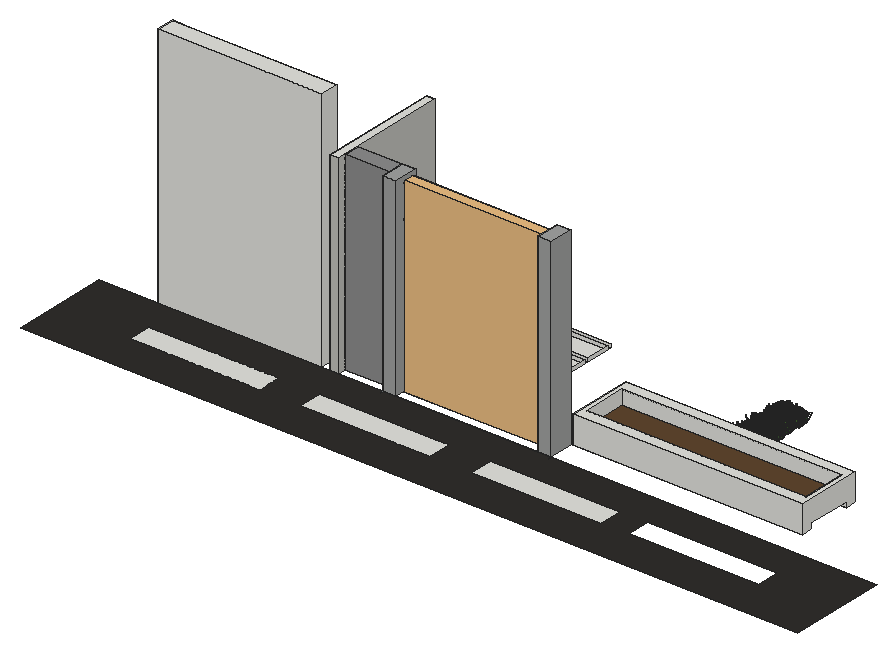
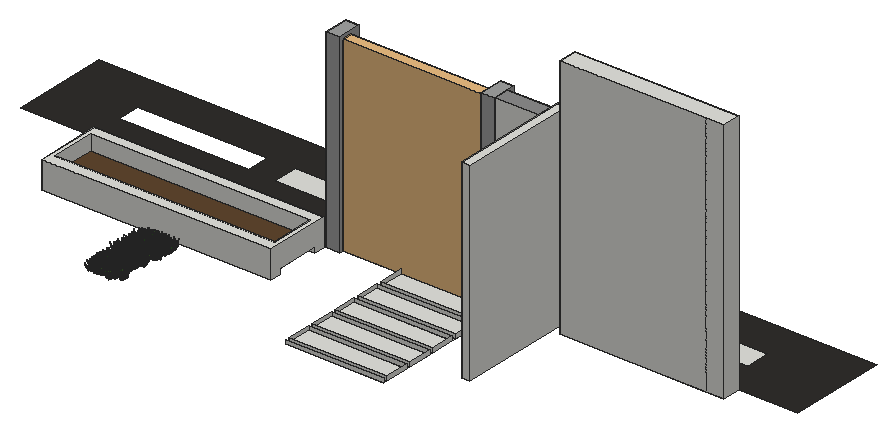
# SketchUp Ruby script. Lengths in inches.
U = 1.inch
M = Sketchup.active_model
def pt(a) = Geom::Point3d.new(a.map { |v| v * U })
def face(e, loops, mat)
  f = e.add_face(loops[0].map { |a| pt(a) })
  loops[1..].each { |l| e.add_face(l.map { |a| pt(a) }).erase! }
  f.material = f.back_material = mat if mat
  f
end
# faces: each face lists its corners as indices into pts; further lists are holes
def faces(e, pts, list, mat = nil) = list.each { |f| face(e, (f[0].is_a?(Array) ? f : [f]).map { |l| l.map { |i| pts[i] } }, mat) }
# xy, xz, yz: faces in a plane at the given z, y or x. An outline is a flat list of corners, or four numbers for a rectangle; further outlines are holes
def ring(l) = l.size == 4 ? [[l[0], l[1]], [l[2], l[1]], [l[2], l[3]], [l[0], l[3]]] : l.each_slice(2).to_a
def flat(e, list, mat, &to3) = list.each { |f| face(e, (f[0].is_a?(Array) ? f : [f]).map { |l| ring(l).map { |u, v| to3.(u, v) } }, mat) }
def xy(e, z, list, mat = nil) = flat(e, list, mat) { |x, y| [x, y, z] }
def xz(e, y, list, mat = nil) = flat(e, list, mat) { |x, z| [x, y, z] }
def yz(e, x, list, mat = nil) = flat(e, list, mat) { |y, z| [x, y, z] }
def lines(e, pts, list) = list.each { |a, b| e.add_line(pt(pts[a]), pt(pts[b])) }
# prism: a flat outline (further loops are holes) pulled along v
def prism(e, loops, v, mat = nil)
  f = face(e, loops, mat); d = Geom::Vector3d.new(v.map { |x| x * U })
  f.pushpull(f.normal.samedirection?(d) ? d.length : -d.length)
end
def box(e, o, s, mat = nil) = prism(e, [[o, [o[0] + s[0], o[1], o[2]], [o[0] + s[0], o[1] + s[1], o[2]], [o[0], o[1] + s[1], o[2]]]], [0, 0, s[2]], mat)
def at(x, y, z, deg = 0) = Geom::Transformation.translation(pt([x, y, z])) * Geom::Transformation.rotation(ORIGIN, Z_AXIS, deg.degrees)
def axes(o, x, y, z) = Geom::Transformation.new([*x, 0, *y, 0, *z, 0, *pt(o).to_a, 1])
def part(name) = M.definitions.add(name)
# library, detail: a bought-in or finely detailed component or shape, given as its bounding box
def library(name, o, s) = part(name).tap { |d| box(d.entities, o, s) }
def detail(e, o, s) = box(e.add_group.entities, o, s)
def put(e, d, t, mat = nil) = e.add_instance(d, t).tap { |i| i.material = mat if mat }
def group(e, t, mat = nil) = e.add_group.tap { |g| g.transformation = t; g.material = mat if mat }.entities
root = M.entities
M.materials.add("18776129-polished-granite-texture-in-whites-grays-and-blacks").color = [192, 192, 186]
M.materials.add("Lisanne_Eraser").color = [146, 152, 155]
M.materials.add("Material1").color = [58, 110, 58]
M.materials.add("Material10").color = [48, 100, 38]
M.materials.add("Material3").color = [68, 110, 58]
M.materials.add("Material4").color = [48, 90, 38]
M.materials.add("Material5").color = [68, 110, 48]
M.materials.add("Material6").color = [48, 90, 48]
M.materials.add("Material8").color = [58, 90, 38]
M.materials.add("Material9").color = [68, 100, 58]
M.materials.add("Material__1").color = [95, 70, 46]
M.materials.add("Stone_A_200cmgach trang tri").color = [160, 161, 160]
M.materials.add("ThomThom - Hat1").color = [48, 46, 44]
M.materials.add("da-to-ong-xam").color = [140, 140, 140]
c1 = part("Group\#69")
xy(c1.entities,0,[[0,0,48,2]])
c2 = library("Group\#91",[0,0,0],[127.95,5.19,98.43])
c3 = part("grass00")
p = [[-0.6875,0.15,0],[-0.56,0.08,5.52],[-0.04,0.03,2.76],[0.48,-0.02,0],[0.35,-0.02,5.52],[-0.1,-0.14,5.52],
  [-0.12,0.65,8.37],[-0.42,0.65,8.37]]
faces(c3.entities,p,[[0,1,2,3],[3,2,4],[1,5,2],[5,4,2],[1,6,5],[4,5,6],[7,6,1]])
c4 = part("Group16\#1")
put(c4.entities,c3,axes([1.44,-0.61,-0.01],[0.05352,0.12609,0],[-0.10704,0.04543,0.07239],[0.06664,-0.02828,0.11628]),"Material6")
put(c4.entities,c3,axes([0.76,-0.15,-0.01],[0.04676,0.24062,0],[-0.23162,0.04501,0.06642],[0.0652,-0.01267,0.23595]),"Material3")
put(c4.entities,c3,axes([0.79,0.01,-0.01],[-0.00606,0.34651,0],[-0.34381,-0.00602,0.0432],[0.04319,0.00076,0.34386]))
put(c4.entities,c3,axes([1,0.23,-0.01],[-0.07192,0.31144,0],[-0.28722,-0.06632,0.1236],[0.12043,0.02781,0.29478]),"Material5")
put(c4.entities,c3,axes([1.66,0.77,-0.01],[-0.13828,0.29651,0],[-0.21551,-0.1005,0.22471],[0.20365,0.09498,0.23779]),"Material10")
put(c4.entities,c3,axes([0.6875,0.52,-0.01],[-0.18126,0.24051,0],[-0.22746,-0.17142,0.09788],[0.07817,0.05891,0.28481]),"Material5")
put(c4.entities,c3,axes([0.68,0.78,-0.01],[-0.215,0.18688,0],[-0.12385,-0.14248,0.21334],[0.13995,0.16101,0.18878]),"Material3")
put(c4.entities,c3,axes([0.56,1,-0.01],[-0.13756,0.07624,0],[-0.06159,-0.11112,0.0927],[0.04494,0.08108,0.12705]),"Material5")
put(c4.entities,c3,axes([0.2,0.64,-0.01],[-0.23729,0.07254,0],[-0.05711,-0.18681,0.153],[0.04473,0.14632,0.19535]),"Material10")
put(c4.entities,c3,axes([0.0625,0.72,-0.01],[-0.28874,0.02525,0],[-0.02179,-0.24916,0.14647],[0.01276,0.14591,0.25012]),"Material3")
put(c4.entities,c3,axes([-0.08,0.62,-0.01],[-0.34089,-0.04187,0],[0.03255,-0.26504,0.216],[-0.02633,0.21439,0.26703]),"Material10")
put(c4.entities,c3,axes([-0.34,0.98,-0.01],[-0.14314,-0.0493,0],[0.04397,-0.12769,0.06843],[-0.02228,0.0647,0.13505]),"Material10")
put(c4.entities,c3,axes([-0.87,1.45,-0.01],[-0.23488,-0.14114,0],[0.13761,-0.22901,0.06087],[-0.03135,0.05217,0.26717]))
put(c4.entities,c3,axes([-0.72,0.77,-0.01],[-0.14208,-0.13251,0],[0.07209,-0.0773,0.16301],[-0.11118,0.11922,0.1057]),"Material10")
put(c4.entities,c3,axes([-0.62,0.43,-0.01],[-0.14845,-0.21203,0],[0.18654,-0.13061,0.12304],[-0.10079,0.07057,0.22772]),"Material3")
put(c4.entities,c3,axes([-0.68,0.29,-0.01],[-0.13639,-0.32136,0],[0.31723,-0.13464,0.05579],[-0.05136,0.0218,0.34462]),"Material4")
put(c4.entities,c3,axes([-0.64,0.125,-0.01],[-0.0458,-0.23569,0],[0.22124,-0.043,0.08276],[-0.08124,0.01579,0.22538]),"Material1")
put(c4.entities,c3,axes([-1.6,-0.03,-0.01],[0.00576,-0.32897,0],[0.27526,0.00482,0.18018],[-0.18015,-0.00315,0.2753]),"Material5")
put(c4.entities,c3,axes([-1.36,-0.31,-0.01],[0.05718,-0.24765,0],[0.18172,0.04196,0.17267],[-0.16825,-0.03885,0.1865]),"Material10")
put(c4.entities,c3,axes([-1.54,-0.72,-0.01],[0.06537,-0.14017,0],[0.13555,0.06321,0.03939],[-0.0357,-0.01665,0.14956]))
put(c4.entities,c3,axes([-1.19,-0.9,-0.01],[0.09597,-0.12735,0],[0.11214,0.08451,0.07557],[-0.06035,-0.04548,0.14042]),"Material9")
put(c4.entities,c3,axes([-0.47,-0.54,-0.01],[0.11588,-0.10072,0],[0.0618,0.0711,0.12124],[-0.07953,-0.0915,0.0942]))
put(c4.entities,c3,axes([-0.47,-0.84,-0.01],[0.11927,-0.0661,0],[0.06603,0.11913,0.00646],[-0.00313,-0.00565,0.13621]),"Material5")
put(c4.entities,c3,axes([-0.38,-1.24,-0.01],[0.28037,-0.08571,0],[0.0618,0.20215,0.20315],[-0.05939,-0.19428,0.21139]),"Material9")
put(c4.entities,c3,axes([-0.06,-0.66,-0.01],[0.22719,-0.01987,0],[0.01247,0.14255,0.17758],[-0.01547,-0.17691,0.1431]),"Material8")
put(c4.entities,c3,axes([0.11,-0.89,-0.01],[0.14882,0.01828,0],[-0.01058,0.08611,0.12229],[0.01491,-0.12138,0.08676]),"Material6")
put(c4.entities,c3,axes([0.25,-0.72,-0.01],[0.20481,0.07053,0],[-0.06206,0.18022,0.10291],[0.03351,-0.0973,0.1906]),"Material6")
put(c4.entities,c3,axes([0.85,-1.42,-0.01],[0.16481,0.09904,0],[-0.09472,0.15762,0.05616],[0.02893,-0.04814,0.18389]),"Material5")
put(c4.entities,c3,axes([1.01,-1.09,-0.01],[0.21858,0.20385,0],[-0.17495,0.1876,0.15339],[0.10462,-0.11218,0.25652]),"Material10")
put(c4.entities,c3,axes([1.01,-0.71,-0.01],[0.08733,0.12473,0],[-0.06445,0.04512,0.13037],[0.1068,-0.07477,0.07867]),"Material6")
c5 = part("Group15\#1")
put(c5.entities,c4,at(0,0,0))
c6 = part("3darcstudiotree_grass00\#1")
put(c6.entities,c5,at(0,0,0))
xy(root,0,[[38.03,19.38,101.65,31.39],[121.5,19.38,185.12,31.39],[205.3,19.38,268.91,31.39],[138.47,57,186.47,70.5],[138.47,72.5,186.47,84.5],
  [138.47,86.5,186.47,98.5],[138.47,100.5,186.47,112.5],[138.47,114.5,186.47,126.5]])
xy(root,0,[[[0,0,380.77,48],[282.38,19.38,346,31.39],[38.03,19.38,101.65,31.39],[205.3,19.38,268.91,31.39],[121.5,19.38,185.12,31.39]]],"ThomThom - Hat1")
xz(root,57,[[138.47,0,186.47,2]])
xz(root,70.5,[[138.47,0,186.47,2]])
xz(root,72.5,[[138.47,0,186.47,2]])
xz(root,84.5,[[138.47,0,186.47,2]])
xz(root,86.5,[[138.47,0,186.47,2]])
xz(root,98.5,[[138.47,0,186.47,2]])
xz(root,100.5,[[138.47,0,186.47,2]])
xz(root,112.5,[[138.47,0,186.47,2]])
xz(root,114.5,[[138.47,0,186.47,2]])
xz(root,126.5,[[138.47,0,186.47,2]])
xz(root,128.5,[[138.47,0,186.47,2]])
yz(root,138.47,[[57,0,70.5,2],[72.5,0,84.5,2],[86.5,0,98.5,2],[100.5,0,112.5,2],[114.5,0,126.5,2]])
yz(root,186.47,[[57,0,70.5,2],[72.5,0,84.5,2],[86.5,0,98.5,2],[100.5,0,112.5,2],[114.5,0,126.5,2]])
g1 = group(root,at(28.97,48,0))
prism(g1,[[[80.27,0,0],[0,0,0],[0,9,0],[9,9,0],[80.27,9,0]]],[0,0,120])
g2 = group(root,at(117.55,38.91,0))
xy(g2,0,[[-4.33,9.09,0,68.14]])
xy(g2,94.52,[[-4.33,9.09,0,68.14]])
xz(g2,9.09,[[-4.33,0,0,94.52]],"18776129-polished-granite-texture-in-whites-grays-and-blacks")
xz(g2,68.14,[[-4.33,0,0,94.52]])
yz(g2,-4.33,[[9.09,0,68.14,94.52]])
yz(g2,0,[[9.09,0,68.14,94.52]],"18776129-polished-granite-texture-in-whites-grays-and-blacks")
g3 = group(root,at(113.14,51.9375,0))
xy(g3,0,[[4.41,0,26.06,7.875]])
xy(g3,94.52,[[4.41,0,26.06,7.875]],"da-to-ong-xam")
xz(g3,0,[[4.41,0,26.06,94.52]],"da-to-ong-xam")
xz(g3,7.875,[[4.41,0,26.06,94.52]])
yz(g3,4.41,[[0,0,7.875,94.52]])
yz(g3,26.06,[[0,0,7.875,94.52]],"da-to-ong-xam")
g4 = group(root,at(139.2,48,0))
box(g4,[0,0,0],[6.5,11.8125,94.52],"Stone_A_200cmgach trang tri")
put(root,c1,at(138.47,70.5,0))
put(root,c1,at(138.47,84.5,0))
put(root,c1,at(138.47,98.5,0))
put(root,c1,at(138.47,112.5,0))
put(root,c1,at(138.47,126.5,0))
put(root,c2,axes([145.7,52.72,0],[0.54154,0,0],[0,1,0],[0,0,0.94148]))
g5 = group(root,at(221.49,28.31,-5.91),"18776129-polished-granite-texture-in-whites-grays-and-blacks")
prism(g5,[[[-82.28,19.69,5.91],[-82.28,19.69,0],[-82.28,0,0]]],[82.28,0,0],"Lisanne_Eraser")
g6 = group(root,at(215,48,0))
box(g6,[0,0,0],[6.5,11.8125,94.52],"Stone_A_200cmgach trang tri")
put(root,c6,axes([266.53,107.4375,0.25],[-0.36611,-0.81728,0],[1.13341,-0.34977,-0.02925],[0.03864,-0.01193,1.7044]))
put(root,c6,axes([266.54,100.88,0.25],[-1.20682,-0.38178,0],[0.32912,-0.7167,-0.04688],[0.02872,-0.06254,1.58936]))
put(root,c6,axes([266.58,103.64,0.25],[0.88864,-0.11909,0],[0.157,0.80706,-0.03713],[0.00837,0.04303,1.39317]))
put(root,c6,axes([266.65,98.22,0.25],[0.41253,0.94156,0],[-0.88752,0.26788,-0.03897],[-0.05944,0.01794,1.53286]))
put(root,c6,axes([267.2,127.18,0.25],[0.10019,-0.95693,0],[1.12696,0.08129,-0.03115],[0.04308,0.00311,1.5702]))
put(root,c6,axes([267.41,98.56,0.25],[0.62314,-0.5766,0],[0.91802,0.68347,-0.03873],[0.04441,0.03306,1.89965]))
put(root,c6,axes([267.57,99.75,0.25],[0.05467,0.83408,0],[-0.92305,0.04168,-0.03311],[-0.05171,0.00233,1.44579]))
put(root,c6,axes([268.02,108.37,0.25],[0.92312,-0.46473,0],[0.65541,0.89686,-0.03972],[0.0268,0.03667,1.6444]))
put(root,c6,axes([267.87,114.85,0.25],[1.00545,0.57433,0],[-0.66851,0.80623,-0.05897],[-0.0542,0.06537,1.91169]))
put(root,c6,axes([268.71,124.54,0.25],[-0.27963,-0.92599,0],[0.92014,-0.19142,-0.0349],[0.06576,-0.01368,1.84282]))
put(root,c6,axes([269.09,117.43,0.25],[-0.62229,-0.66442,0],[0.79434,-0.51252,-0.04864],[0.07207,-0.0465,1.88819]))
put(root,c6,axes([269.08,106.91,0.25],[-0.0748,-0.80388,0],[1.10854,-0.07106,-0.04603],[0.06655,-0.00427,1.61216]))
put(root,c6,axes([269.22,118.81,0.25],[-1.15837,-0.11855,0],[0.12341,-0.83068,-0.03319],[0.00626,-0.04216,1.55524]))
put(root,c6,axes([269.3,126.83,0.25],[-0.36924,-0.87792,0],[1.16903,-0.33871,-0.05387],[0.06012,-0.01742,1.46363]))
put(root,c6,axes([268.93,112.01,0.25],[0.97613,-0.075,0],[0.10315,0.92487,-0.05657],[0.00697,0.06249,1.49576]))
put(root,c6,axes([269.36,120.625,0.25],[-0.85959,-0.43604,0],[0.55383,-0.75214,-0.04274],[0.03488,-0.04737,1.66217]))
put(root,c6,axes([269.16,121.99,0.25],[-0.1699,0.87577,0],[-0.987,-0.13191,-0.03829],[-0.06433,-0.0086,1.70109]))
put(root,c6,axes([269.65,110.03,0.25],[-1.1904,-0.1584,0],[0.17094,-0.885,-0.05495],[0.01293,-0.06695,1.60563]))
put(root,c6,axes([269.29,108.68,0.25],[0.48534,0.7559,0],[-0.8924,0.39473,-0.05193],[-0.084,0.03715,1.85357]))
put(root,c6,axes([269.71,119.18,0.25],[0.14475,-0.84801,0],[0.96208,0.11313,-0.02485],[0.04999,0.00588,1.97391]))
put(root,c6,axes([269.7,100.67,0.25],[-0.46242,0.98987,0],[-1.09288,-0.35172,-0.03012],[-0.04366,-0.01405,1.82227]))
put(root,c6,axes([269.66,125.71,0.25],[0.71999,0.56892,0],[-0.74106,0.64608,-0.04733],[-0.04003,0.0349,1.31836]))
put(root,c6,axes([269.76,104.11,0.25],[0.67082,0.87639,0],[-0.86854,0.45799,-0.05376],[-0.07483,0.03946,1.69687]))
put(root,c6,axes([270.29,101.9375,0.25],[-0.87308,-0.57881,0],[0.59112,-0.61425,-0.04095],[0.04754,-0.0494,1.76156]))
put(root,c6,axes([270.39,121.09,0.25],[-0.39323,0.91693,0],[-1.04934,-0.31002,-0.05045],[-0.06966,-0.02058,1.63245]))
put(root,c6,axes([270.29,122.04,0.25],[0.49527,0.87719,0],[-0.9516,0.37013,-0.0367],[-0.06302,0.02451,1.99296]))
put(root,c6,axes([270.7,98.33,0.25],[-0.90026,-0.03545,0],[0.04766,-0.83381,-0.03298],[0.00292,-0.05106,1.87797]))
put(root,c6,axes([270.74,127.12,0.25],[-0.10693,-0.88747,0],[1.14044,-0.09467,-0.04439],[0.05374,-0.00446,1.39437]))
put(root,c6,axes([270.53,126.26,0.25],[1.13537,-0.29522,0],[0.35727,0.94654,-0.0458],[0.02034,0.0539,1.7756]))
put(root,c6,axes([270.44,100.3,0.25],[0.89738,0.77477,0],[-0.69052,0.55098,-0.03508],[-0.04224,0.03371,1.59982]))
put(root,c6,axes([270.75,99.23,0.25],[0.61887,-0.73613,0],[0.87976,0.50953,-0.05108],[0.06998,0.04053,1.79238]))
put(root,c6,axes([270.88,128.35,0.25],[0.81927,-0.75327,0],[0.94118,0.70518,-0.0538],[0.04323,0.03239,1.37259]))
put(root,c6,axes([271.02,108.06,0.25],[-0.73545,0.70435,0],[-0.79172,-0.5695,-0.03703],[-0.04244,-0.03053,1.58908]))
put(root,c6,axes([270.8125,123.16,0.25],[0.29469,0.82661,0],[-1.15482,0.28362,-0.04809],[-0.05235,0.01286,1.36712]))
put(root,c6,axes([270.88,129.8,0.25],[0.36261,0.87726,0],[-1.12778,0.32114,-0.02597],[-0.04052,0.01154,1.96681]))
put(root,c6,axes([271.78,122.08,0.25],[-0.86837,-0.20995,0],[0.35566,-1.01338,-0.03129],[0.01269,-0.03616,1.8441]))
put(root,c6,axes([272.08,100.64,0.25],[-0.74474,-0.58215,0],[0.79932,-0.70444,-0.03536],[0.03744,-0.033,1.8008]))
put(root,c6,axes([271.9,129.76,0.25],[-0.56257,0.69066,0],[-0.82158,-0.46102,-0.04556],[-0.07449,-0.0418,1.95702]))
put(root,c6,axes([271.79,116.91,0.25],[-0.23219,0.82133,0],[-1.08812,-0.21191,-0.03302],[-0.04332,-0.00844,1.5061]))
put(root,c6,axes([272.16,99.94,0.25],[0.47608,-0.98921,0],[0.97172,0.32217,-0.05078],[0.07787,0.02582,1.72798]))
put(root,c6,axes([272.6,102.84,0.25],[-0.44555,-0.67696,0],[1.01055,-0.4582,-0.05959],[0.05927,-0.02687,1.30502]))
put(root,c6,axes([272.39,119.62,0.25],[0.48587,-0.66924,0],[0.78414,0.39218,-0.04784],[0.07795,0.03899,1.7418]))
put(root,c6,axes([272.24,118.59,0.25],[0.06095,0.98404,0],[-1.15392,0.04924,-0.0387],[-0.05728,0.00244,1.71236]))
put(root,c6,axes([272.2,111.94,0.25],[0.38517,0.85107,0],[-1.20109,0.37447,-0.05425],[-0.06826,0.02128,1.72469]))
put(root,c6,axes([272.3125,128.64,0.25],[1.02446,-0.23604,0],[0.2807,0.83929,-0.05393],[0.02492,0.07452,1.81331]))
put(root,c6,axes([272.51,107.32,0.25],[-0.26049,1.00552,0],[-1.01434,-0.18102,-0.03186],[-0.05881,-0.0105,1.95913]))
put(root,c6,axes([272.8,126.05,0.25],[0.8939,-0.23665,0],[0.38058,0.99035,-0.05774],[0.02678,0.06968,1.91123]))
put(root,c6,axes([273.5,105.78,0.25],[-0.59526,-0.75678,0],[1.07721,-0.58371,-0.04707],[0.04267,-0.02312,1.39282]))
put(root,c6,axes([273.4,100.71,0.25],[-0.91845,0.0591,0],[-0.07951,-0.85127,-0.03359],[-0.00494,-0.05293,1.95875]))
put(root,c6,axes([273.25,98.62,0.25],[1.07415,-0.22114,0],[0.28161,0.94235,-0.04456],[0.01316,0.04403,1.43455]))
put(root,c6,axes([273.66,112.03,0.25],[0.16473,-0.79509,0],[1.06351,0.1518,-0.05034],[0.0815,0.01163,1.77282]))
put(root,c6,axes([273.48,99.53,0.25],[1.07708,-0.51717,0],[0.54613,0.78355,-0.042],[0.03013,0.04323,1.56273]))
put(root,c6,axes([273.53,128.13,0.25],[-0.30421,0.75295,0],[-0.90762,-0.25262,-0.03292],[-0.06313,-0.01757,1.93659]))
put(root,c6,axes([273.9,119.45,0.25],[-0.41802,-0.76273,0],[0.87616,-0.3308,-0.03768],[0.06314,-0.02384,1.77164]))
put(root,c6,axes([273.65,122.56,0.25],[-0.28373,0.82686,0],[-1.1161,-0.26383,-0.05457],[-0.06239,-0.01475,1.37935]))
put(root,c6,axes([273.99,123.43,0.25],[-0.97851,-0.0019,0],[0.00256,-0.90826,-0.04252],[0.00016,-0.05539,1.71753]))
put(root,c6,axes([273.91,121.28,0.25],[0.40125,-0.99259,0],[1.10477,0.30766,-0.04434],[0.06977,0.01943,1.93394]))
put(root,c6,axes([273.72,126.7,0.25],[0.23434,0.77393,0],[-1.20276,0.25089,-0.04255],[-0.05214,0.01088,1.5668]))
put(root,c6,axes([273.78,116.73,0.25],[-0.02429,0.84379,0],[-1.11846,-0.02218,-0.0357],[-0.04578,-0.00091,1.43525]))
put(root,c6,axes([273.96,109.14,0.25],[-0.42223,0.88893,0],[-1.08477,-0.35496,-0.03242],[-0.0508,-0.01662,1.96368]))
put(root,c6,axes([274.33,108.02,0.25],[-1.11166,-0.17426,0],[0.23308,-1.02429,-0.03943],[0.00941,-0.04134,1.61444]))
put(root,c6,axes([274.15,113.59,0.25],[1.2429,0.12136,0],[-0.13564,0.95697,-0.02625],[-0.0052,0.03667,1.96735]))
put(root,c6,axes([274.8125,119.39,0.25],[0.55005,-0.62458,0],[1.00138,0.60753,-0.0361],[0.04236,0.0257,1.80295]))
put(root,c6,axes([274.89,113.76,0.25],[1.03554,-0.11533,0],[0.13808,0.85407,-0.04419],[0.0085,0.05259,1.50171]))
put(root,c6,axes([274.85,98.41,0.25],[0.86607,0.26447,0],[-0.41488,0.93595,-0.05896],[-0.03292,0.07428,1.94308]))
put(root,c6,axes([275.17,128.3,0.25],[0.21479,-0.90594,0],[1.05964,0.17308,-0.05061],[0.08971,0.01465,1.95081]))
put(root,c6,axes([275.32,116.0625,0.25],[-1.16516,0.02645,0],[-0.02981,-0.90472,-0.04984],[-0.00187,-0.0567,1.49526]))
put(root,c6,axes([275.32,116.77,0.25],[0.18176,-0.86146,0],[1.25226,0.18202,-0.04237],[0.06339,0.00921,1.93074]))
put(root,c6,axes([275.1875,107.95,0.25],[-0.33314,0.92343,0],[-0.88891,-0.22092,-0.04102],[-0.07073,-0.01758,1.67021]))
put(root,c6,axes([275.5,129.625,0.25],[0.44312,-0.69577,0],[1.09117,0.47875,-0.05061],[0.07089,0.0311,1.95538]))
put(root,c6,axes([275.71,99.23,0.25],[-1.20386,-0.24079,0],[0.26585,-0.91568,-0.03666],[0.00985,-0.03393,1.30149]))
put(root,c6,axes([275.75,121.98,0.25],[0.25938,-0.81974,0],[1.0212,0.2226,-0.03356],[0.04953,0.0108,1.61101]))
put(root,c6,axes([275.47,104.5,0.25],[1.09163,-0.08679,0],[0.09738,0.84381,-0.02913],[0.00541,0.04691,1.9903]))
put(root,c6,axes([275.84,114.53,0.25],[0.03091,-1.05851,0],[1.23997,0.02495,-0.04883],[0.06274,0.00126,1.59403]))
put(root,c6,axes([276.26,106.68,0.25],[0.7004,-0.63696,0],[0.88144,0.6677,-0.03913],[0.03756,0.02845,1.55084]))
put(root,c6,axes([276.45,116.96,0.25],[-1.27532,0.20066,0],[-0.20513,-0.89815,-0.04366],[-0.01262,-0.05525,1.70895]))
put(root,c6,axes([276.63,123.35,0.25],[-0.98615,-0.41616,0],[0.4496,-0.73395,-0.05096],[0.03742,-0.06108,1.60728]))
put(root,c6,axes([276.67,128.43,0.25],[0.54303,-0.62632,0],[1.02426,0.61178,-0.05142],[0.06528,0.03899,1.97373]))
put(root,c6,axes([276.42,110.9,0.25],[0.54151,0.63482,0],[-0.95081,0.55874,-0.06047],[-0.05683,0.0334,1.34144]))
put(root,c6,axes([276.66,116.11,0.25],[0.81336,-0.36743,0],[0.48428,0.73852,-0.04084],[0.03742,0.05707,1.94165]))
put(root,c6,axes([277.1,118.45,0.25],[-0.74751,-0.469,0],[0.69817,-0.76658,-0.03674],[0.03101,-0.03405,1.62045]))
put(root,c6,axes([276.79,126.78,0.25],[0.95194,-0.16617,0],[0.24214,0.95565,-0.04208],[0.00983,0.0388,1.3356]))
put(root,c6,axes([276.76,98.69,0.25],[0.87025,0.61618,0],[-0.81316,0.79117,-0.05603],[-0.05213,0.05072,1.79617]))
put(root,c6,axes([277.22,121.26,0.25],[0.42581,-0.87959,0],[1.16747,0.38935,-0.03894],[0.05616,0.01873,1.95573]))
put(root,c6,axes([277.14,97.34,0.25],[1.02597,0.281,0],[-0.28779,0.72386,-0.0401],[-0.02313,0.05817,1.69032]))
put(root,c6,axes([277.79,118.57,0.25],[-1.24669,0.16028,0],[-0.18553,-0.9941,-0.03016],[-0.0062,-0.03321,1.62739]))
put(root,c6,axes([277.9,98.05,0.25],[-0.93361,0.19141,0],[-0.23759,-0.79835,-0.03348],[-0.01232,-0.0414,1.52035]))
put(root,c6,axes([278.42,104.64,0.25],[-0.26521,-0.97797,0],[1.09294,-0.20418,-0.03143],[0.04181,-0.00781,1.52743]))
put(root,c6,axes([278.46,126.82,0.25],[-0.94687,-0.17816,0],[0.23955,-0.87706,-0.03754],[0.01489,-0.0545,1.94323]))
put(root,c6,axes([278.38,105.41,0.25],[-0.12034,-0.92052,0],[0.96781,-0.08716,-0.05057],[0.0917,-0.00826,1.77563]))
g7 = group(root,at(222.18,93.1,0))
xy(g7,0,[[0,-32.4,112.21,-27],[0,-5.4,112.21,0]])
xy(g7,2.7,[[0,-27,112.21,-5.4]])
xy(g7,6.3,[[2.39,-27,109.82,-5.4]],"Material__1")
xy(g7,13.5,[[[0,-32.4,112.21,0],[2.39,-27,109.82,-5.4]]])
xz(g7,-32.4,[[0,0,112.21,13.5]])
xz(g7,-27,[[0,0,112.21,2.7],[2.39,6.3,109.82,13.5]])
xz(g7,-5.4,[[0,0,112.21,2.7],[2.39,6.3,109.82,13.5]])
xz(g7,0,[[0,0,112.21,13.5]])
yz(g7,0,[[-32.4,0,-32.4,13.5,0,13.5,0,0,-5.4,0,-5.4,2.7,-27,2.7,-27,0]])
yz(g7,2.39,[[-27,6.3,-5.4,13.5]])
yz(g7,109.82,[[-27,6.3,-5.4,13.5]])
yz(g7,112.21,[[-32.4,0,-27,0,-27,2.7,-5.4,2.7,-5.4,0,0,0,0,13.5,-32.4,13.5]])
put(root,c6,axes([278.1,113.32,0.25],[0.84498,0.38162,0],[-0.48332,0.73723,-0.04213],[-0.02702,0.04121,1.35679]))
put(root,c6,axes([278.39,129.44,0.25],[1.07604,0.0041,0],[-0.00425,0.76772,-0.03904],[-0.00036,0.06489,1.85207]))
put(root,c6,axes([278.67,107.85,0.25],[0.54025,-0.97959,0],[0.93471,0.35512,-0.04178],[0.06001,0.0228,1.62381]))
put(root,c6,axes([278.44,115.44,0.25],[0.905,0.533,0],[-0.69587,0.81396,-0.05586],[-0.04108,0.04805,1.52805]))
put(root,c6,axes([278.69,124.72,0.25],[0.84802,-0.25454,0],[0.38277,0.87851,-0.04794],[0.01972,0.04526,1.36124]))
put(root,c6,axes([278.89,123.84,0.25],[0.82019,-0.45453,0],[0.66712,0.82932,-0.03164],[0.0278,0.03455,1.90074]))
put(root,c6,axes([278.85,120.58,0.25],[1.21755,-0.30605,0],[0.34631,0.9491,-0.03542],[0.01238,0.03392,1.44036]))
put(root,c6,axes([279.29,124.71,0.25],[0.65398,-0.51729,0],[0.65362,0.56927,-0.03437],[0.04176,0.03637,1.66865]))
put(root,c6,axes([279.92,100.68,0.25],[-0.86474,-0.22191,0],[0.3457,-0.92803,-0.02785],[0.01276,-0.03424,1.81462]))
put(root,c6,axes([279.74,103.35,0.25],[-0.41423,0.69811,0],[-0.91992,-0.37603,-0.03193],[-0.04752,-0.01942,1.70102]))
put(root,c6,axes([280.05,107.03,0.25],[-1.02756,0.07402,0],[-0.07851,-0.75081,-0.03872],[-0.00659,-0.063,1.78675]))
put(root,c6,axes([279.71,129.63,0.25],[0.90167,0.3279,0],[-0.51111,0.96822,-0.0492],[-0.02394,0.04535,1.54416]))
put(root,c6,axes([279.79,104.51,0.25],[0.88078,0.23536,0],[-0.31812,0.82012,-0.048],[-0.02605,0.06717,1.83855]))
put(root,c6,axes([280.18,125.85,0.25],[0.27271,-0.71311,0],[1.21971,0.32133,-0.04397],[0.04693,0.01236,1.43296]))
put(root,c6,axes([280.07,114.16,0.25],[1.01596,-0.52557,0],[0.57998,0.77236,-0.04378],[0.03788,0.05045,1.79394]))
put(root,c6,axes([279.95,109.65,0.25],[0.20256,0.91819,0],[-1.21747,0.18503,-0.04305],[-0.06259,0.00951,1.82947]))
put(root,c6,axes([280.08,111.875,0.25],[0.15897,1.02035,0],[-1.06955,0.1148,-0.04685],[-0.07217,0.00775,1.67517]))
put(root,c6,axes([280.4,119.43,0.25],[0.28155,-0.75657,0],[0.92644,0.23751,-0.03395],[0.05048,0.01294,1.50895]))
